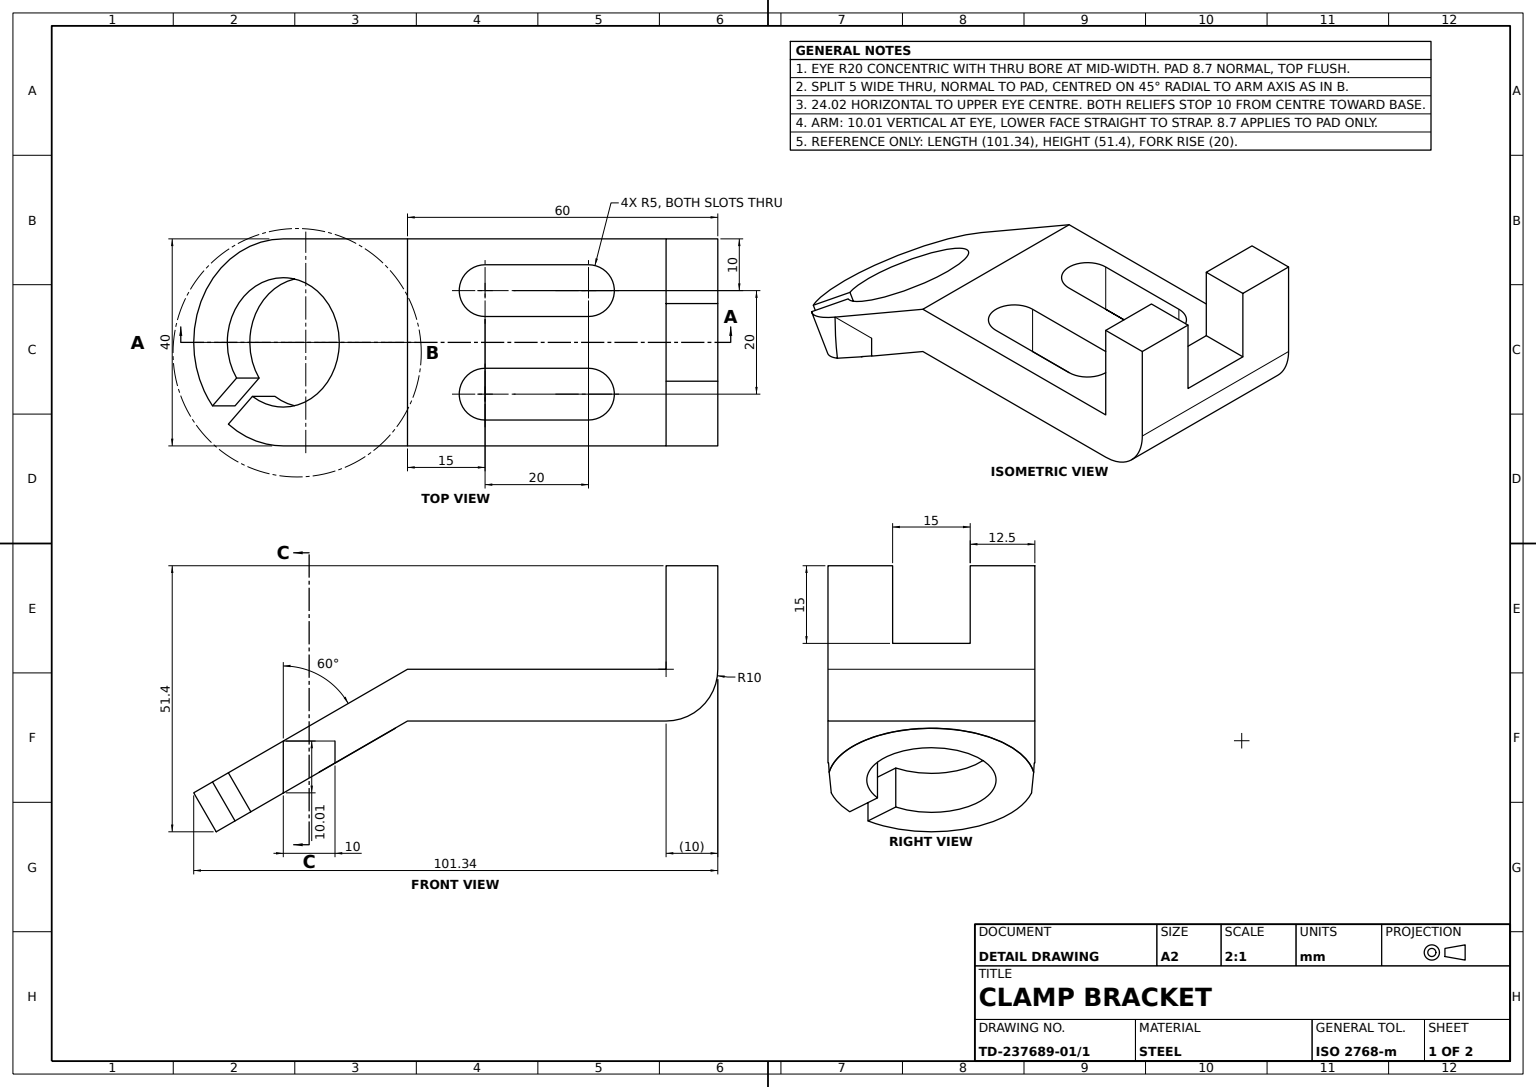
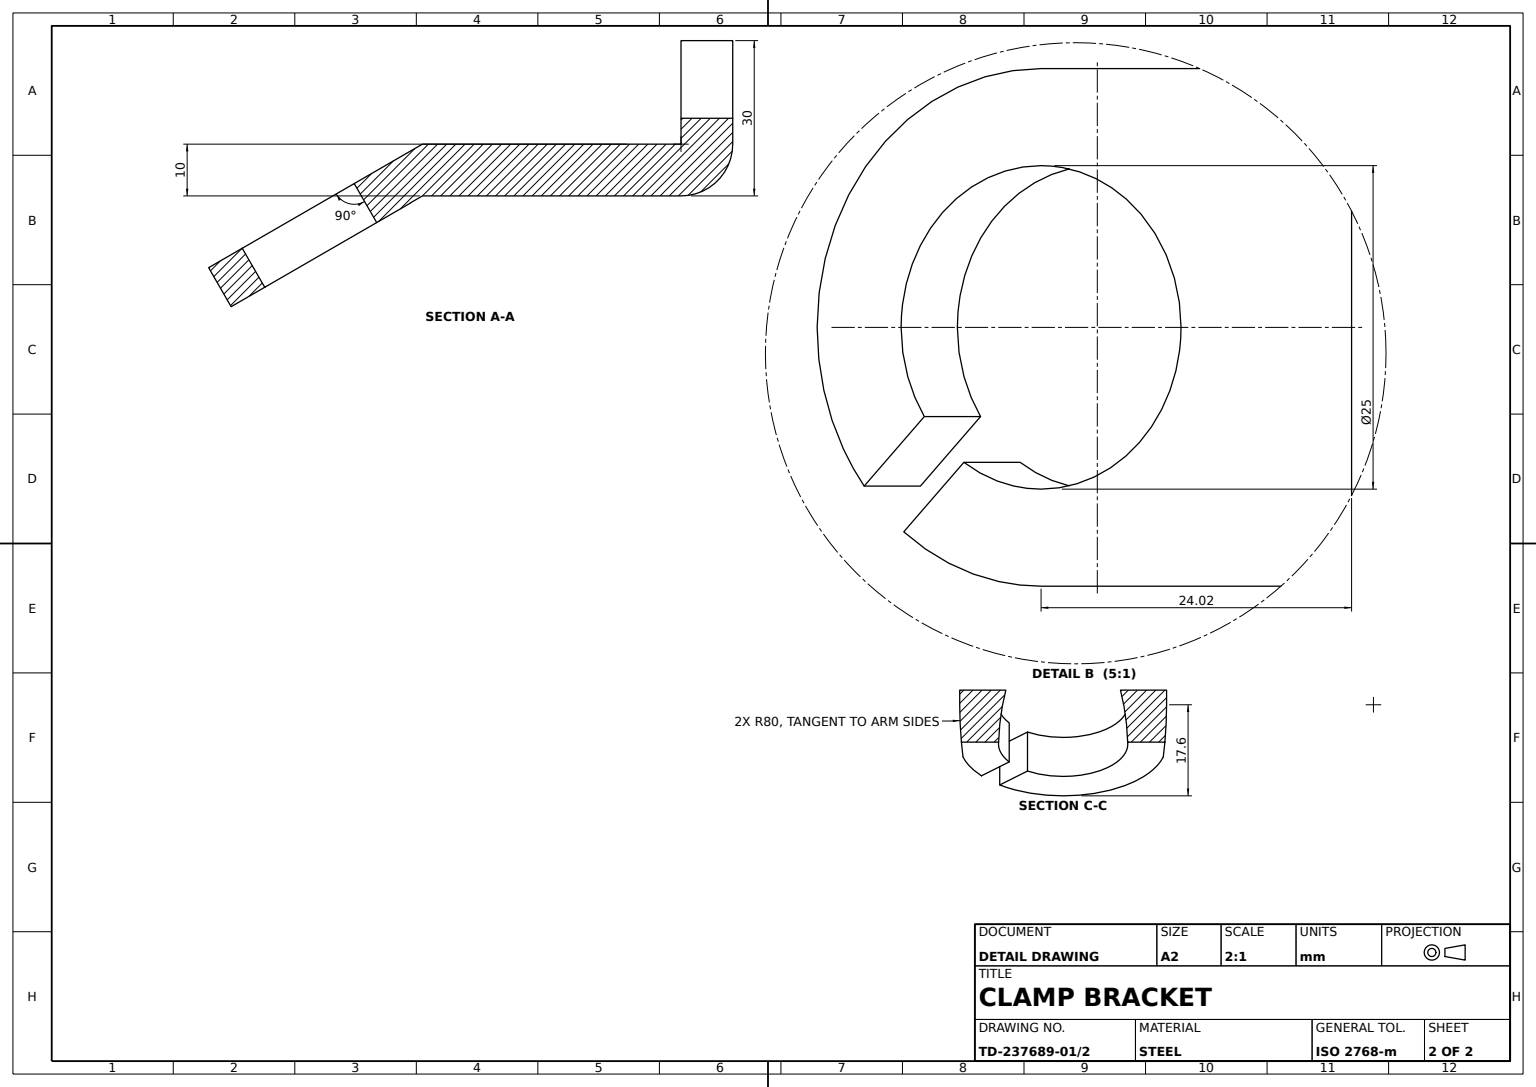
ISO-10303-21;
HEADER;
FILE_DESCRIPTION((''),'2;1');
FILE_NAME('','',(''),(''),'','','');
FILE_SCHEMA(('AUTOMOTIVE_DESIGN'));
ENDSEC;
DATA;
#1=APPLICATION_CONTEXT('');
#2=PRODUCT_CONTEXT('',#1,'mechanical');
#3=PRODUCT('','','',(#2));
#4=PRODUCT_DEFINITION_FORMATION('','',#3);
#5=PRODUCT_DEFINITION_CONTEXT('',#1,'design');
#6=PRODUCT_DEFINITION('','',#4,#5);
#7=PRODUCT_DEFINITION_SHAPE('','',#6);
#8=(LENGTH_UNIT()NAMED_UNIT(*)SI_UNIT(.MILLI.,.METRE.));
#9=(NAMED_UNIT(*)PLANE_ANGLE_UNIT()SI_UNIT($,.RADIAN.));
#10=(NAMED_UNIT(*)SI_UNIT($,.STERADIAN.)SOLID_ANGLE_UNIT());
#11=UNCERTAINTY_MEASURE_WITH_UNIT(LENGTH_MEASURE(1.E-05),#8,'distance_accuracy_value','');
#12=(GEOMETRIC_REPRESENTATION_CONTEXT(3)GLOBAL_UNCERTAINTY_ASSIGNED_CONTEXT((#11))GLOBAL_UNIT_ASSIGNED_CONTEXT((#8,#9,#10))REPRESENTATION_CONTEXT('',''));
#13=CARTESIAN_POINT('',(60.,30.,-27.5));
#14=VERTEX_POINT('',#13);
#15=CARTESIAN_POINT('',(50.,30.,-27.5));
#16=VERTEX_POINT('',#15);
#17=CARTESIAN_POINT('',(90.,30.,-27.5));
#18=DIRECTION('',(-1.,0.,0.));
#19=VECTOR('',#18,1000.);
#20=LINE('',#17,#19);
#21=EDGE_CURVE('',#14,#16,#20,.T.);
#22=ORIENTED_EDGE('',*,*,#21,.F.);
#23=CARTESIAN_POINT('',(60.,30.,-40.));
#24=VERTEX_POINT('',#23);
#25=DIRECTION('',(0.,0.,1.));
#26=VECTOR('',#25,1000.);
#27=LINE('',#23,#26);
#28=EDGE_CURVE('',#24,#14,#27,.T.);
#29=ORIENTED_EDGE('',*,*,#28,.F.);
#30=CARTESIAN_POINT('',(50.,30.,-40.));
#31=VERTEX_POINT('',#30);
#32=LINE('',#23,#19);
#33=EDGE_CURVE('',#24,#31,#32,.T.);
#34=ORIENTED_EDGE('',*,*,#33,.T.);
#35=LINE('',#30,#26);
#36=EDGE_CURVE('',#31,#16,#35,.T.);
#37=ORIENTED_EDGE('',*,*,#36,.T.);
#38=EDGE_LOOP('',(#22,#29,#34,#37));
#39=FACE_OUTER_BOUND('',#38,.T.);
#40=DIRECTION('',(0.,1.,0.));
#41=AXIS2_PLACEMENT_3D('',#23,#40,#25);
#42=PLANE('',#41);
#43=ADVANCED_FACE('',(#39),#42,.T.);
#44=CARTESIAN_POINT('',(60.,30.,-12.5));
#45=VERTEX_POINT('',#44);
#46=CARTESIAN_POINT('',(60.,15.,-12.5));
#47=VERTEX_POINT('',#46);
#48=CARTESIAN_POINT('',(60.,10.,-12.5));
#49=DIRECTION('',(0.,-1.,0.));
#50=VECTOR('',#49,1000.);
#51=LINE('',#48,#50);
#52=EDGE_CURVE('',#45,#47,#51,.T.);
#53=ORIENTED_EDGE('',*,*,#52,.T.);
#54=CARTESIAN_POINT('',(50.,15.,-12.5));
#55=VERTEX_POINT('',#54);
#56=CARTESIAN_POINT('',(90.,15.,-12.5));
#57=LINE('',#56,#19);
#58=EDGE_CURVE('',#47,#55,#57,.T.);
#59=ORIENTED_EDGE('',*,*,#58,.T.);
#60=CARTESIAN_POINT('',(50.,30.,-12.5));
#61=VERTEX_POINT('',#60);
#62=VECTOR('',#40,1000.);
#63=LINE('',#54,#62);
#64=EDGE_CURVE('',#55,#61,#63,.T.);
#65=ORIENTED_EDGE('',*,*,#64,.T.);
#66=CARTESIAN_POINT('',(90.,30.,-12.5));
#67=LINE('',#66,#19);
#68=EDGE_CURVE('',#45,#61,#67,.T.);
#69=ORIENTED_EDGE('',*,*,#68,.F.);
#70=EDGE_LOOP('',(#53,#59,#65,#69));
#71=FACE_OUTER_BOUND('',#70,.T.);
#72=DIRECTION('',(1.,0.,0.));
#73=AXIS2_PLACEMENT_3D('',#56,#25,#72);
#74=PLANE('',#73);
#75=ADVANCED_FACE('',(#71),#74,.F.);
#76=CARTESIAN_POINT('',(-17.067657,-9.860231,-39.770555));
#77=VERTEX_POINT('',#76);
#78=CARTESIAN_POINT('',(-17.040219,-9.88407,-39.768742));
#79=VERTEX_POINT('',#78);
#80=CARTESIAN_POINT('',(-17.058511,-9.868177,-39.769952));
#81=CARTESIAN_POINT('',(-17.049365,-9.876123,-39.769348));
#82=B_SPLINE_CURVE_WITH_KNOTS('',3,(#76,#80,#81,#78),.UNSPECIFIED.,.F.,.F.,(4,4),(0.00917853,0.009214903),.UNSPECIFIED.);
#83=EDGE_CURVE('',#77,#79,#82,.T.);
#84=ORIENTED_EDGE('',*,*,#83,.F.);
#85=CARTESIAN_POINT('',(-17.067657,-9.860231,-0.229445));
#86=VERTEX_POINT('',#85);
#87=CARTESIAN_POINT('',(8.925723,5.156518,-4.816157));
#88=CARTESIAN_POINT('',(8.925723,5.156518,-35.183843));
#89=(BOUNDED_CURVE()B_SPLINE_CURVE(3,(#85,#87,#88,#76),.UNSPECIFIED.,.F.,.T.)B_SPLINE_CURVE_WITH_KNOTS((4,4),(4.864008458,7.702362156),.UNSPECIFIED.)CURVE()GEOMETRIC_REPRESENTATION_ITEM()RATIONAL_B_SPLINE_CURVE((1.,0.434026152,0.434026152,1.))REPRESENTATION_ITEM(''));
#90=EDGE_CURVE('',#86,#77,#89,.T.);
#91=ORIENTED_EDGE('',*,*,#90,.F.);
#92=CARTESIAN_POINT('',(-17.040219,-9.88407,-0.231258));
#93=VERTEX_POINT('',#92);
#94=CARTESIAN_POINT('',(-17.049365,-9.876123,-0.230652));
#95=CARTESIAN_POINT('',(-17.058511,-9.868177,-0.230048));
#96=B_SPLINE_CURVE_WITH_KNOTS('',3,(#92,#94,#95,#85),.UNSPECIFIED.,.F.,.F.,(4,4),(0.,0.00003639),.UNSPECIFIED.);
#97=EDGE_CURVE('',#93,#86,#96,.T.);
#98=ORIENTED_EDGE('',*,*,#97,.F.);
#99=CARTESIAN_POINT('',(-19.666551,-11.400383,-20.));
#100=DIRECTION('',(-0.5,0.866025404,0.));
#101=DIRECTION('',(-0.866025404,-0.5,0.));
#102=AXIS2_PLACEMENT_3D('',#99,#100,#101);
#103=CIRCLE('',#102,20.);
#104=EDGE_CURVE('',#93,#79,#103,.T.);
#105=ORIENTED_EDGE('',*,*,#104,.T.);
#106=EDGE_LOOP('',(#84,#91,#98,#105));
#107=FACE_OUTER_BOUND('',#106,.T.);
#108=CYLINDRICAL_SURFACE('',#102,20.);
#109=ADVANCED_FACE('',(#107),#108,.T.);
#110=CARTESIAN_POINT('',(50.,30.,0.));
#111=VERTEX_POINT('',#110);
#112=EDGE_CURVE('',#61,#111,#35,.T.);
#113=ORIENTED_EDGE('',*,*,#112,.F.);
#114=ORIENTED_EDGE('',*,*,#64,.F.);
#115=CARTESIAN_POINT('',(50.,15.,-27.5));
#116=VERTEX_POINT('',#115);
#117=LINE('',#115,#26);
#118=EDGE_CURVE('',#116,#55,#117,.T.);
#119=ORIENTED_EDGE('',*,*,#118,.F.);
#120=LINE('',#15,#50);
#121=EDGE_CURVE('',#16,#116,#120,.T.);
#122=ORIENTED_EDGE('',*,*,#121,.F.);
#123=ORIENTED_EDGE('',*,*,#36,.F.);
#124=CARTESIAN_POINT('',(50.,10.,-40.));
#125=VERTEX_POINT('',#124);
#126=LINE('',#124,#50);
#127=EDGE_CURVE('',#31,#125,#126,.T.);
#128=ORIENTED_EDGE('',*,*,#127,.T.);
#129=CARTESIAN_POINT('',(50.,10.,0.));
#130=VERTEX_POINT('',#129);
#131=LINE('',#124,#26);
#132=EDGE_CURVE('',#125,#130,#131,.T.);
#133=ORIENTED_EDGE('',*,*,#132,.T.);
#134=LINE('',#129,#50);
#135=EDGE_CURVE('',#111,#130,#134,.T.);
#136=ORIENTED_EDGE('',*,*,#135,.F.);
#137=EDGE_LOOP('',(#113,#114,#119,#122,#123,#128,#133,#136));
#138=FACE_OUTER_BOUND('',#137,.T.);
#139=AXIS2_PLACEMENT_3D('',#124,#18,#25);
#140=PLANE('',#139);
#141=ADVANCED_FACE('',(#138),#140,.T.);
#142=CARTESIAN_POINT('',(-23.952204,-13.874706,-39.363787));
#143=VERTEX_POINT('',#142);
#144=CARTESIAN_POINT('',(-24.016551,-13.874706,-39.363787));
#145=VERTEX_POINT('',#144);
#146=CARTESIAN_POINT('',(-14.016551,-13.874706,-39.363787));
#147=LINE('',#146,#19);
#148=EDGE_CURVE('',#143,#145,#147,.T.);
#149=ORIENTED_EDGE('',*,*,#148,.F.);
#150=CARTESIAN_POINT('',(-23.952204,-13.874706,-39.378104));
#151=VERTEX_POINT('',#150);
#152=CARTESIAN_POINT('',(-23.952204,-13.874706,-20.));
#153=LINE('',#152,#26);
#154=EDGE_CURVE('',#151,#143,#153,.T.);
#155=ORIENTED_EDGE('',*,*,#154,.F.);
#156=CARTESIAN_POINT('',(-23.973661,-13.874706,-39.373358));
#157=CARTESIAN_POINT('',(-23.99511,-13.874706,-39.368586));
#158=(BOUNDED_CURVE()B_SPLINE_CURVE(3,(#150,#156,#157,#144),.UNSPECIFIED.,.F.,.T.)B_SPLINE_CURVE_WITH_KNOTS((4,4),(4.962418222,4.965295009),.UNSPECIFIED.)CURVE()GEOMETRIC_REPRESENTATION_ITEM()RATIONAL_B_SPLINE_CURVE((1.,0.99999931,0.99999931,1.))REPRESENTATION_ITEM(''));
#159=EDGE_CURVE('',#151,#145,#158,.T.);
#160=ORIENTED_EDGE('',*,*,#159,.T.);
#161=EDGE_LOOP('',(#149,#155,#160));
#162=FACE_OUTER_BOUND('',#161,.T.);
#163=CARTESIAN_POINT('',(-14.016551,-13.874706,-40.));
#164=DIRECTION('',(0.,0.,-1.));
#165=AXIS2_PLACEMENT_3D('',#163,#49,#164);
#166=PLANE('',#165);
#167=ADVANCED_FACE('',(#162),#166,.F.);
#168=CARTESIAN_POINT('',(-24.016551,-3.865962,-40.));
#169=VERTEX_POINT('',#168);
#170=CARTESIAN_POINT('',(-24.016551,-10.556136,-39.784836));
#171=CARTESIAN_POINT('',(-24.016551,-7.211136,-39.997464));
#172=B_SPLINE_CURVE_WITH_KNOTS('',3,(#144,#170,#171,#168),.UNSPECIFIED.,.F.,.F.,(4,4),(0.,1.),.UNSPECIFIED.);
#173=EDGE_CURVE('',#145,#169,#172,.T.);
#174=ORIENTED_EDGE('',*,*,#173,.T.);
#175=CARTESIAN_POINT('',(-14.016551,-3.865962,-40.));
#176=VERTEX_POINT('',#175);
#177=LINE('',#175,#19);
#178=EDGE_CURVE('',#176,#169,#177,.T.);
#179=ORIENTED_EDGE('',*,*,#178,.F.);
#180=CARTESIAN_POINT('',(-14.016551,-8.097563,-39.884793));
#181=VERTEX_POINT('',#180);
#182=CARTESIAN_POINT('',(-14.016551,-3.805302,39.999977));
#183=AXIS2_PLACEMENT_3D('',#182,#72,#164);
#184=CIRCLE('',#183,80.);
#185=EDGE_CURVE('',#181,#176,#184,.T.);
#186=ORIENTED_EDGE('',*,*,#185,.F.);
#187=CARTESIAN_POINT('',(-16.05137,-9.273107,-39.815121));
#188=CARTESIAN_POINT('',(-15.034294,-8.685527,-39.853201));
#189=(BOUNDED_CURVE()B_SPLINE_CURVE(3,(#76,#187,#188,#180),.UNSPECIFIED.,.F.,.T.)B_SPLINE_CURVE_WITH_KNOTS((4,4),(1.49503727,1.51711729),.UNSPECIFIED.)CURVE()GEOMETRIC_REPRESENTATION_ITEM()RATIONAL_B_SPLINE_CURVE((1.,0.999959373,0.999959373,1.))REPRESENTATION_ITEM(''));
#190=EDGE_CURVE('',#77,#181,#189,.T.);
#191=ORIENTED_EDGE('',*,*,#190,.F.);
#192=ORIENTED_EDGE('',*,*,#83,.T.);
#193=CARTESIAN_POINT('',(-21.654313,-12.548018,-39.532113));
#194=CARTESIAN_POINT('',(-19.349835,-11.217527,-39.667126));
#195=(BOUNDED_CURVE()B_SPLINE_CURVE(3,(#142,#193,#194,#78),.UNSPECIFIED.,.F.,.T.)B_SPLINE_CURVE_WITH_KNOTS((4,4),(1.444594034,1.494738419),.UNSPECIFIED.)CURVE()GEOMETRIC_REPRESENTATION_ITEM()RATIONAL_B_SPLINE_CURVE((1.,0.999790473,0.999790473,1.))REPRESENTATION_ITEM(''));
#196=EDGE_CURVE('',#143,#79,#195,.T.);
#197=ORIENTED_EDGE('',*,*,#196,.F.);
#198=ORIENTED_EDGE('',*,*,#148,.T.);
#199=EDGE_LOOP('',(#174,#179,#186,#191,#192,#197,#198));
#200=FACE_OUTER_BOUND('',#199,.T.);
#201=AXIS2_PLACEMENT_3D('',#182,#18,#25);
#202=CYLINDRICAL_SURFACE('',#201,80.);
#203=ADVANCED_FACE('',(#200),#202,.T.);
#204=CARTESIAN_POINT('',(35.,10.,-25.));
#205=VERTEX_POINT('',#204);
#206=CARTESIAN_POINT('',(35.,10.,-35.));
#207=VERTEX_POINT('',#206);
#208=CARTESIAN_POINT('',(35.,10.,-30.));
#209=AXIS2_PLACEMENT_3D('',#208,#40,#25);
#210=CIRCLE('',#209,5.);
#211=EDGE_CURVE('',#205,#207,#210,.T.);
#212=ORIENTED_EDGE('',*,*,#211,.T.);
#213=CARTESIAN_POINT('',(35.,0.,-35.));
#214=VERTEX_POINT('',#213);
#215=LINE('',#213,#62);
#216=EDGE_CURVE('',#214,#207,#215,.T.);
#217=ORIENTED_EDGE('',*,*,#216,.F.);
#218=CARTESIAN_POINT('',(35.,0.,-25.));
#219=VERTEX_POINT('',#218);
#220=CARTESIAN_POINT('',(35.,0.,-30.));
#221=AXIS2_PLACEMENT_3D('',#220,#40,#25);
#222=CIRCLE('',#221,5.);
#223=EDGE_CURVE('',#219,#214,#222,.T.);
#224=ORIENTED_EDGE('',*,*,#223,.F.);
#225=LINE('',#218,#62);
#226=EDGE_CURVE('',#219,#205,#225,.T.);
#227=ORIENTED_EDGE('',*,*,#226,.T.);
#228=EDGE_LOOP('',(#212,#217,#224,#227));
#229=FACE_OUTER_BOUND('',#228,.T.);
#230=CYLINDRICAL_SURFACE('',#221,5.);
#231=ADVANCED_FACE('',(#229),#230,.F.);
#232=CARTESIAN_POINT('',(-33.348871,-19.299874,-7.736552));
#233=VERTEX_POINT('',#232);
#234=CARTESIAN_POINT('',(-37.698871,-11.765453,-7.736552));
#235=VERTEX_POINT('',#234);
#236=CARTESIAN_POINT('',(-32.698871,-20.425707,-7.736552));
#237=VECTOR('',#100,1000.);
#238=LINE('',#236,#237);
#239=EDGE_CURVE('',#233,#235,#238,.T.);
#240=ORIENTED_EDGE('',*,*,#239,.F.);
#241=CARTESIAN_POINT('',(-28.697482,-16.614394,-13.107513));
#242=VERTEX_POINT('',#241);
#243=CARTESIAN_POINT('',(-21.197482,-12.284267,-21.767767));
#244=DIRECTION('',(-0.612372436,-0.353553391,0.707106781));
#245=VECTOR('',#244,1000.);
#246=LINE('',#243,#245);
#247=EDGE_CURVE('',#242,#233,#246,.T.);
#248=ORIENTED_EDGE('',*,*,#247,.F.);
#249=CARTESIAN_POINT('',(-33.047482,-9.079973,-13.107513));
#250=VERTEX_POINT('',#249);
#251=CARTESIAN_POINT('',(-28.047482,-17.740227,-13.107513));
#252=LINE('',#251,#237);
#253=EDGE_CURVE('',#242,#250,#252,.T.);
#254=ORIENTED_EDGE('',*,*,#253,.T.);
#255=LINE('',#234,#245);
#256=EDGE_CURVE('',#250,#235,#255,.T.);
#257=ORIENTED_EDGE('',*,*,#256,.T.);
#258=EDGE_LOOP('',(#240,#248,#254,#257));
#259=FACE_OUTER_BOUND('',#258,.T.);
#260=DIRECTION('',(-0.612372436,-0.353553391,-0.707106781));
#261=DIRECTION('',(-0.755928946,0.,0.654653671));
#262=AXIS2_PLACEMENT_3D('',#236,#260,#261);
#263=PLANE('',#262);
#264=ADVANCED_FACE('',(#259),#263,.F.);
#265=CARTESIAN_POINT('',(15.,10.,-5.));
#266=VERTEX_POINT('',#265);
#267=CARTESIAN_POINT('',(35.,10.,-5.));
#268=VERTEX_POINT('',#267);
#269=CARTESIAN_POINT('',(0.,10.,-5.));
#270=VECTOR('',#72,1000.);
#271=LINE('',#269,#270);
#272=EDGE_CURVE('',#266,#268,#271,.T.);
#273=ORIENTED_EDGE('',*,*,#272,.F.);
#274=CARTESIAN_POINT('',(15.,10.,-15.));
#275=VERTEX_POINT('',#274);
#276=CARTESIAN_POINT('',(15.,10.,-10.));
#277=AXIS2_PLACEMENT_3D('',#276,#40,#25);
#278=CIRCLE('',#277,5.);
#279=EDGE_CURVE('',#275,#266,#278,.T.);
#280=ORIENTED_EDGE('',*,*,#279,.F.);
#281=CARTESIAN_POINT('',(35.,10.,-15.));
#282=VERTEX_POINT('',#281);
#283=CARTESIAN_POINT('',(0.,10.,-15.));
#284=LINE('',#283,#270);
#285=EDGE_CURVE('',#275,#282,#284,.T.);
#286=ORIENTED_EDGE('',*,*,#285,.T.);
#287=CARTESIAN_POINT('',(35.,10.,-10.));
#288=AXIS2_PLACEMENT_3D('',#287,#40,#25);
#289=CIRCLE('',#288,5.);
#290=EDGE_CURVE('',#268,#282,#289,.T.);
#291=ORIENTED_EDGE('',*,*,#290,.F.);
#292=EDGE_LOOP('',(#273,#280,#286,#291));
#293=FACE_BOUND('',#292,.T.);
#294=ORIENTED_EDGE('',*,*,#132,.F.);
#295=CARTESIAN_POINT('',(0.,10.,-40.));
#296=VERTEX_POINT('',#295);
#297=LINE('',#295,#19);
#298=EDGE_CURVE('',#125,#296,#297,.T.);
#299=ORIENTED_EDGE('',*,*,#298,.T.);
#300=CARTESIAN_POINT('',(0.,10.,0.));
#301=VERTEX_POINT('',#300);
#302=LINE('',#295,#26);
#303=EDGE_CURVE('',#296,#301,#302,.T.);
#304=ORIENTED_EDGE('',*,*,#303,.T.);
#305=LINE('',#300,#19);
#306=EDGE_CURVE('',#130,#301,#305,.T.);
#307=ORIENTED_EDGE('',*,*,#306,.F.);
#308=EDGE_LOOP('',(#294,#299,#304,#307));
#309=FACE_OUTER_BOUND('',#308,.T.);
#310=ORIENTED_EDGE('',*,*,#211,.F.);
#311=CARTESIAN_POINT('',(15.,10.,-25.));
#312=VERTEX_POINT('',#311);
#313=CARTESIAN_POINT('',(0.,10.,-25.));
#314=LINE('',#313,#270);
#315=EDGE_CURVE('',#312,#205,#314,.T.);
#316=ORIENTED_EDGE('',*,*,#315,.F.);
#317=CARTESIAN_POINT('',(15.,10.,-35.));
#318=VERTEX_POINT('',#317);
#319=CARTESIAN_POINT('',(15.,10.,-30.));
#320=AXIS2_PLACEMENT_3D('',#319,#40,#25);
#321=CIRCLE('',#320,5.);
#322=EDGE_CURVE('',#318,#312,#321,.T.);
#323=ORIENTED_EDGE('',*,*,#322,.F.);
#324=CARTESIAN_POINT('',(0.,10.,-35.));
#325=LINE('',#324,#270);
#326=EDGE_CURVE('',#318,#207,#325,.T.);
#327=ORIENTED_EDGE('',*,*,#326,.T.);
#328=EDGE_LOOP('',(#310,#316,#323,#327));
#329=FACE_BOUND('',#328,.T.);
#330=AXIS2_PLACEMENT_3D('',#295,#40,#25);
#331=PLANE('',#330);
#332=ADVANCED_FACE('',(#293,#309,#329),#331,.T.);
#333=CARTESIAN_POINT('',(15.,0.,-15.));
#334=VERTEX_POINT('',#333);
#335=CARTESIAN_POINT('',(35.,0.,-15.));
#336=VERTEX_POINT('',#335);
#337=CARTESIAN_POINT('',(0.,0.,-15.));
#338=LINE('',#337,#270);
#339=EDGE_CURVE('',#334,#336,#338,.T.);
#340=ORIENTED_EDGE('',*,*,#339,.T.);
#341=LINE('',#335,#62);
#342=EDGE_CURVE('',#336,#282,#341,.T.);
#343=ORIENTED_EDGE('',*,*,#342,.T.);
#344=ORIENTED_EDGE('',*,*,#285,.F.);
#345=LINE('',#333,#62);
#346=EDGE_CURVE('',#334,#275,#345,.T.);
#347=ORIENTED_EDGE('',*,*,#346,.F.);
#348=EDGE_LOOP('',(#340,#343,#344,#347));
#349=FACE_OUTER_BOUND('',#348,.T.);
#350=AXIS2_PLACEMENT_3D('',#337,#25,#72);
#351=PLANE('',#350);
#352=ADVANCED_FACE('',(#349),#351,.T.);
#353=CARTESIAN_POINT('',(-34.637009,-9.997687,-4.201018));
#354=VERTEX_POINT('',#353);
#355=CARTESIAN_POINT('',(-24.016551,-3.865962,0.));
#356=VERTEX_POINT('',#355);
#357=CARTESIAN_POINT('',(-24.016551,-3.865962,-20.));
#358=AXIS2_PLACEMENT_3D('',#357,#100,#101);
#359=CIRCLE('',#358,20.);
#360=EDGE_CURVE('',#354,#356,#359,.T.);
#361=ORIENTED_EDGE('',*,*,#360,.F.);
#362=CARTESIAN_POINT('',(-30.287009,-17.532108,-4.201018));
#363=VERTEX_POINT('',#362);
#364=CARTESIAN_POINT('',(-29.637009,-18.657941,-4.201018));
#365=LINE('',#364,#237);
#366=EDGE_CURVE('',#363,#354,#365,.T.);
#367=ORIENTED_EDGE('',*,*,#366,.F.);
#368=CARTESIAN_POINT('',(-23.952204,-13.874706,-0.621896));
#369=VERTEX_POINT('',#368);
#370=EDGE_CURVE('',#363,#369,#103,.T.);
#371=ORIENTED_EDGE('',*,*,#370,.T.);
#372=CARTESIAN_POINT('',(-24.016551,-13.874706,-0.636213));
#373=VERTEX_POINT('',#372);
#374=CARTESIAN_POINT('',(-23.99511,-13.874706,-0.631414));
#375=CARTESIAN_POINT('',(-23.973661,-13.874706,-0.626642));
#376=(BOUNDED_CURVE()B_SPLINE_CURVE(3,(#372,#374,#375,#368),.UNSPECIFIED.,.F.,.T.)B_SPLINE_CURVE_WITH_KNOTS((4,4),(1.317890298,1.320767086),.UNSPECIFIED.)CURVE()GEOMETRIC_REPRESENTATION_ITEM()RATIONAL_B_SPLINE_CURVE((1.,0.99999931,0.99999931,1.))REPRESENTATION_ITEM(''));
#377=EDGE_CURVE('',#373,#369,#376,.T.);
#378=ORIENTED_EDGE('',*,*,#377,.F.);
#379=CARTESIAN_POINT('',(-24.016551,-7.211136,-0.002536));
#380=CARTESIAN_POINT('',(-24.016551,-10.556136,-0.215164));
#381=B_SPLINE_CURVE_WITH_KNOTS('',3,(#355,#379,#380,#372),.UNSPECIFIED.,.F.,.F.,(4,4),(0.,1.),.UNSPECIFIED.);
#382=EDGE_CURVE('',#356,#373,#381,.T.);
#383=ORIENTED_EDGE('',*,*,#382,.F.);
#384=EDGE_LOOP('',(#361,#367,#371,#378,#383));
#385=FACE_OUTER_BOUND('',#384,.T.);
#386=ADVANCED_FACE('',(#385),#108,.T.);
#387=ORIENTED_EDGE('',*,*,#366,.T.);
#388=CARTESIAN_POINT('',(-29.98562,-7.312206,-9.571979));
#389=VERTEX_POINT('',#388);
#390=DIRECTION('',(0.612372436,0.353553391,-0.707106781));
#391=VECTOR('',#390,1000.);
#392=LINE('',#388,#391);
#393=EDGE_CURVE('',#354,#389,#392,.T.);
#394=ORIENTED_EDGE('',*,*,#393,.T.);
#395=CARTESIAN_POINT('',(-25.63562,-14.846627,-9.571979));
#396=VERTEX_POINT('',#395);
#397=CARTESIAN_POINT('',(-24.98562,-15.97246,-9.571979));
#398=LINE('',#397,#237);
#399=EDGE_CURVE('',#396,#389,#398,.T.);
#400=ORIENTED_EDGE('',*,*,#399,.F.);
#401=CARTESIAN_POINT('',(-18.13562,-10.5165,-18.232233));
#402=LINE('',#401,#391);
#403=EDGE_CURVE('',#363,#396,#402,.T.);
#404=ORIENTED_EDGE('',*,*,#403,.F.);
#405=EDGE_LOOP('',(#387,#394,#400,#404));
#406=FACE_OUTER_BOUND('',#405,.T.);
#407=DIRECTION('',(0.612372436,0.353553391,0.707106781));
#408=DIRECTION('',(0.755928946,0.,-0.654653671));
#409=AXIS2_PLACEMENT_3D('',#397,#407,#408);
#410=PLANE('',#409);
#411=ADVANCED_FACE('',(#406),#410,.F.);
#412=CARTESIAN_POINT('',(-30.491869,-17.650383,-20.));
#413=VERTEX_POINT('',#412);
#414=CARTESIAN_POINT('',(-34.841869,-10.115962,-20.));
#415=VERTEX_POINT('',#414);
#416=CARTESIAN_POINT('',(-29.841869,-18.776216,-20.));
#417=LINE('',#416,#237);
#418=EDGE_CURVE('',#413,#415,#417,.T.);
#419=ORIENTED_EDGE('',*,*,#418,.F.);
#420=CARTESIAN_POINT('',(-8.841234,-5.150383,-20.));
#421=VERTEX_POINT('',#420);
#422=CIRCLE('',#102,12.5);
#423=EDGE_CURVE('',#421,#413,#422,.T.);
#424=ORIENTED_EDGE('',*,*,#423,.F.);
#425=CARTESIAN_POINT('',(-13.191234,2.384038,-20.));
#426=VERTEX_POINT('',#425);
#427=CARTESIAN_POINT('',(-8.191234,-6.276216,-20.));
#428=LINE('',#427,#237);
#429=EDGE_CURVE('',#421,#426,#428,.T.);
#430=ORIENTED_EDGE('',*,*,#429,.T.);
#431=CIRCLE('',#358,12.5);
#432=EDGE_CURVE('',#426,#415,#431,.T.);
#433=ORIENTED_EDGE('',*,*,#432,.T.);
#434=EDGE_LOOP('',(#419,#424,#430,#433));
#435=FACE_OUTER_BOUND('',#434,.T.);
#436=CARTESIAN_POINT('',(-19.016551,-12.526216,-20.));
#437=AXIS2_PLACEMENT_3D('',#436,#100,#101);
#438=CYLINDRICAL_SURFACE('',#437,12.5);
#439=ADVANCED_FACE('',(#435),#438,.F.);
#440=CARTESIAN_POINT('',(15.,0.,-5.));
#441=VERTEX_POINT('',#440);
#442=CARTESIAN_POINT('',(15.,0.,-10.));
#443=AXIS2_PLACEMENT_3D('',#442,#40,#25);
#444=CIRCLE('',#443,5.);
#445=EDGE_CURVE('',#334,#441,#444,.T.);
#446=ORIENTED_EDGE('',*,*,#445,.F.);
#447=ORIENTED_EDGE('',*,*,#346,.T.);
#448=ORIENTED_EDGE('',*,*,#279,.T.);
#449=LINE('',#440,#62);
#450=EDGE_CURVE('',#441,#266,#449,.T.);
#451=ORIENTED_EDGE('',*,*,#450,.F.);
#452=EDGE_LOOP('',(#446,#447,#448,#451));
#453=FACE_OUTER_BOUND('',#452,.T.);
#454=CYLINDRICAL_SURFACE('',#443,5.);
#455=ADVANCED_FACE('',(#453),#454,.F.);
#456=ORIENTED_EDGE('',*,*,#377,.T.);
#457=CARTESIAN_POINT('',(-23.952204,-13.874706,-0.636213));
#458=VERTEX_POINT('',#457);
#459=EDGE_CURVE('',#458,#369,#153,.T.);
#460=ORIENTED_EDGE('',*,*,#459,.F.);
#461=CARTESIAN_POINT('',(-14.016551,-13.874706,-0.636213));
#462=LINE('',#461,#19);
#463=EDGE_CURVE('',#458,#373,#462,.T.);
#464=ORIENTED_EDGE('',*,*,#463,.T.);
#465=EDGE_LOOP('',(#456,#460,#464));
#466=FACE_OUTER_BOUND('',#465,.T.);
#467=AXIS2_PLACEMENT_3D('',#461,#49,#164);
#468=PLANE('',#467);
#469=ADVANCED_FACE('',(#466),#468,.F.);
#470=CARTESIAN_POINT('',(60.,30.,0.));
#471=VERTEX_POINT('',#470);
#472=LINE('',#470,#19);
#473=EDGE_CURVE('',#471,#111,#472,.T.);
#474=ORIENTED_EDGE('',*,*,#473,.F.);
#475=EDGE_CURVE('',#45,#471,#27,.T.);
#476=ORIENTED_EDGE('',*,*,#475,.F.);
#477=ORIENTED_EDGE('',*,*,#68,.T.);
#478=ORIENTED_EDGE('',*,*,#112,.T.);
#479=EDGE_LOOP('',(#474,#476,#477,#478));
#480=FACE_OUTER_BOUND('',#479,.T.);
#481=ADVANCED_FACE('',(#480),#42,.T.);
#482=CARTESIAN_POINT('',(-14.016551,-8.097563,0.));
#483=VERTEX_POINT('',#482);
#484=CARTESIAN_POINT('',(-14.016551,-8.097563,-0.115207));
#485=VERTEX_POINT('',#484);
#486=CARTESIAN_POINT('',(-14.016551,-8.097563,-40.));
#487=VECTOR('',#164,1000.);
#488=LINE('',#486,#487);
#489=EDGE_CURVE('',#483,#485,#488,.T.);
#490=ORIENTED_EDGE('',*,*,#489,.T.);
#491=CARTESIAN_POINT('',(-15.034294,-8.685527,-0.146799));
#492=CARTESIAN_POINT('',(-16.05137,-9.273107,-0.184879));
#493=(BOUNDED_CURVE()B_SPLINE_CURVE(3,(#484,#491,#492,#85),.UNSPECIFIED.,.F.,.T.)B_SPLINE_CURVE_WITH_KNOTS((4,4),(4.766068017,4.788148037),.UNSPECIFIED.)CURVE()GEOMETRIC_REPRESENTATION_ITEM()RATIONAL_B_SPLINE_CURVE((1.,0.999959373,0.999959373,1.))REPRESENTATION_ITEM(''));
#494=EDGE_CURVE('',#485,#86,#493,.T.);
#495=ORIENTED_EDGE('',*,*,#494,.T.);
#496=ORIENTED_EDGE('',*,*,#90,.T.);
#497=ORIENTED_EDGE('',*,*,#190,.T.);
#498=VERTEX_POINT('',#486);
#499=EDGE_CURVE('',#181,#498,#488,.T.);
#500=ORIENTED_EDGE('',*,*,#499,.T.);
#501=CARTESIAN_POINT('',(0.,0.,-40.));
#502=VERTEX_POINT('',#501);
#503=DIRECTION('',(-0.865888863,-0.50023642,0.));
#504=VECTOR('',#503,1000.);
#505=LINE('',#501,#504);
#506=EDGE_CURVE('',#502,#498,#505,.T.);
#507=ORIENTED_EDGE('',*,*,#506,.F.);
#508=CARTESIAN_POINT('',(0.,0.,0.));
#509=VERTEX_POINT('',#508);
#510=LINE('',#501,#26);
#511=EDGE_CURVE('',#502,#509,#510,.T.);
#512=ORIENTED_EDGE('',*,*,#511,.T.);
#513=LINE('',#508,#504);
#514=EDGE_CURVE('',#509,#483,#513,.T.);
#515=ORIENTED_EDGE('',*,*,#514,.T.);
#516=EDGE_LOOP('',(#490,#495,#496,#497,#500,#507,#512,#515));
#517=FACE_OUTER_BOUND('',#516,.T.);
#518=DIRECTION('',(-0.50023642,0.865888863,0.));
#519=AXIS2_PLACEMENT_3D('',#501,#518,#503);
#520=PLANE('',#519);
#521=ADVANCED_FACE('',(#517),#520,.F.);
#522=CARTESIAN_POINT('',(35.,0.,-5.));
#523=VERTEX_POINT('',#522);
#524=LINE('',#522,#62);
#525=EDGE_CURVE('',#523,#268,#524,.T.);
#526=ORIENTED_EDGE('',*,*,#525,.F.);
#527=CARTESIAN_POINT('',(0.,0.,-5.));
#528=LINE('',#527,#270);
#529=EDGE_CURVE('',#441,#523,#528,.T.);
#530=ORIENTED_EDGE('',*,*,#529,.F.);
#531=ORIENTED_EDGE('',*,*,#450,.T.);
#532=ORIENTED_EDGE('',*,*,#272,.T.);
#533=EDGE_LOOP('',(#526,#530,#531,#532));
#534=FACE_OUTER_BOUND('',#533,.T.);
#535=AXIS2_PLACEMENT_3D('',#527,#25,#72);
#536=PLANE('',#535);
#537=ADVANCED_FACE('',(#534),#536,.F.);
#538=ORIENTED_EDGE('',*,*,#21,.T.);
#539=ORIENTED_EDGE('',*,*,#121,.T.);
#540=CARTESIAN_POINT('',(60.,15.,-27.5));
#541=VERTEX_POINT('',#540);
#542=CARTESIAN_POINT('',(90.,15.,-27.5));
#543=LINE('',#542,#19);
#544=EDGE_CURVE('',#541,#116,#543,.T.);
#545=ORIENTED_EDGE('',*,*,#544,.F.);
#546=CARTESIAN_POINT('',(60.,10.,-27.5));
#547=LINE('',#546,#62);
#548=EDGE_CURVE('',#541,#14,#547,.T.);
#549=ORIENTED_EDGE('',*,*,#548,.T.);
#550=EDGE_LOOP('',(#538,#539,#545,#549));
#551=FACE_OUTER_BOUND('',#550,.T.);
#552=AXIS2_PLACEMENT_3D('',#17,#164,#18);
#553=PLANE('',#552);
#554=ADVANCED_FACE('',(#551),#553,.F.);
#555=EDGE_CURVE('',#413,#242,#422,.T.);
#556=ORIENTED_EDGE('',*,*,#555,.F.);
#557=ORIENTED_EDGE('',*,*,#418,.T.);
#558=EDGE_CURVE('',#415,#250,#431,.T.);
#559=ORIENTED_EDGE('',*,*,#558,.T.);
#560=ORIENTED_EDGE('',*,*,#253,.F.);
#561=EDGE_LOOP('',(#556,#557,#559,#560));
#562=FACE_OUTER_BOUND('',#561,.T.);
#563=ADVANCED_FACE('',(#562),#438,.F.);
#564=ORIENTED_EDGE('',*,*,#514,.F.);
#565=CARTESIAN_POINT('',(50.,0.,0.));
#566=VERTEX_POINT('',#565);
#567=LINE('',#508,#270);
#568=EDGE_CURVE('',#509,#566,#567,.T.);
#569=ORIENTED_EDGE('',*,*,#568,.T.);
#570=CARTESIAN_POINT('',(60.,10.,0.));
#571=VERTEX_POINT('',#570);
#572=AXIS2_PLACEMENT_3D('',#129,#25,#72);
#573=CIRCLE('',#572,10.);
#574=EDGE_CURVE('',#566,#571,#573,.T.);
#575=ORIENTED_EDGE('',*,*,#574,.T.);
#576=LINE('',#570,#62);
#577=EDGE_CURVE('',#571,#471,#576,.T.);
#578=ORIENTED_EDGE('',*,*,#577,.T.);
#579=ORIENTED_EDGE('',*,*,#473,.T.);
#580=ORIENTED_EDGE('',*,*,#135,.T.);
#581=ORIENTED_EDGE('',*,*,#306,.T.);
#582=CARTESIAN_POINT('',(-4.330127,7.5,0.));
#583=VECTOR('',#101,1000.);
#584=LINE('',#582,#583);
#585=EDGE_CURVE('',#301,#356,#584,.T.);
#586=ORIENTED_EDGE('',*,*,#585,.T.);
#587=CARTESIAN_POINT('',(-14.016551,-3.865962,0.));
#588=VERTEX_POINT('',#587);
#589=LINE('',#587,#19);
#590=EDGE_CURVE('',#588,#356,#589,.T.);
#591=ORIENTED_EDGE('',*,*,#590,.F.);
#592=CARTESIAN_POINT('',(-14.016551,-13.874706,0.));
#593=LINE('',#592,#62);
#594=EDGE_CURVE('',#483,#588,#593,.T.);
#595=ORIENTED_EDGE('',*,*,#594,.F.);
#596=EDGE_LOOP('',(#564,#569,#575,#578,#579,#580,#581,#586,#591,#595));
#597=FACE_OUTER_BOUND('',#596,.T.);
#598=PLANE('',#572);
#599=ADVANCED_FACE('',(#597),#598,.T.);
#600=CARTESIAN_POINT('',(15.,0.,-35.));
#601=VERTEX_POINT('',#600);
#602=CARTESIAN_POINT('',(0.,0.,-35.));
#603=LINE('',#602,#270);
#604=EDGE_CURVE('',#601,#214,#603,.T.);
#605=ORIENTED_EDGE('',*,*,#604,.F.);
#606=CARTESIAN_POINT('',(15.,0.,-25.));
#607=VERTEX_POINT('',#606);
#608=CARTESIAN_POINT('',(15.,0.,-30.));
#609=AXIS2_PLACEMENT_3D('',#608,#40,#25);
#610=CIRCLE('',#609,5.);
#611=EDGE_CURVE('',#601,#607,#610,.T.);
#612=ORIENTED_EDGE('',*,*,#611,.T.);
#613=CARTESIAN_POINT('',(0.,0.,-25.));
#614=LINE('',#613,#270);
#615=EDGE_CURVE('',#607,#219,#614,.T.);
#616=ORIENTED_EDGE('',*,*,#615,.T.);
#617=ORIENTED_EDGE('',*,*,#223,.T.);
#618=EDGE_LOOP('',(#605,#612,#616,#617));
#619=FACE_BOUND('',#618,.T.);
#620=CARTESIAN_POINT('',(35.,0.,-10.));
#621=AXIS2_PLACEMENT_3D('',#620,#40,#25);
#622=CIRCLE('',#621,5.);
#623=EDGE_CURVE('',#523,#336,#622,.T.);
#624=ORIENTED_EDGE('',*,*,#623,.T.);
#625=ORIENTED_EDGE('',*,*,#339,.F.);
#626=ORIENTED_EDGE('',*,*,#445,.T.);
#627=ORIENTED_EDGE('',*,*,#529,.T.);
#628=EDGE_LOOP('',(#624,#625,#626,#627));
#629=FACE_BOUND('',#628,.T.);
#630=CARTESIAN_POINT('',(50.,0.,-40.));
#631=VERTEX_POINT('',#630);
#632=LINE('',#630,#26);
#633=EDGE_CURVE('',#631,#566,#632,.T.);
#634=ORIENTED_EDGE('',*,*,#633,.T.);
#635=ORIENTED_EDGE('',*,*,#568,.F.);
#636=ORIENTED_EDGE('',*,*,#511,.F.);
#637=LINE('',#501,#270);
#638=EDGE_CURVE('',#502,#631,#637,.T.);
#639=ORIENTED_EDGE('',*,*,#638,.T.);
#640=EDGE_LOOP('',(#634,#635,#636,#639));
#641=FACE_OUTER_BOUND('',#640,.T.);
#642=AXIS2_PLACEMENT_3D('',#501,#49,#164);
#643=PLANE('',#642);
#644=ADVANCED_FACE('',(#619,#629,#641),#643,.T.);
#645=CARTESIAN_POINT('',(-41.337059,-13.865962,-20.));
#646=VERTEX_POINT('',#645);
#647=EDGE_CURVE('',#169,#646,#359,.T.);
#648=ORIENTED_EDGE('',*,*,#647,.F.);
#649=ORIENTED_EDGE('',*,*,#173,.F.);
#650=ORIENTED_EDGE('',*,*,#159,.F.);
#651=CARTESIAN_POINT('',(-36.987059,-21.400383,-20.));
#652=VERTEX_POINT('',#651);
#653=EDGE_CURVE('',#151,#652,#103,.T.);
#654=ORIENTED_EDGE('',*,*,#653,.T.);
#655=LINE('',#651,#237);
#656=EDGE_CURVE('',#652,#646,#655,.T.);
#657=ORIENTED_EDGE('',*,*,#656,.T.);
#658=EDGE_LOOP('',(#648,#649,#650,#654,#657));
#659=FACE_OUTER_BOUND('',#658,.T.);
#660=ADVANCED_FACE('',(#659),#108,.T.);
#661=LINE('',#163,#50);
#662=EDGE_CURVE('',#176,#498,#661,.T.);
#663=ORIENTED_EDGE('',*,*,#662,.T.);
#664=ORIENTED_EDGE('',*,*,#499,.F.);
#665=ORIENTED_EDGE('',*,*,#185,.T.);
#666=EDGE_LOOP('',(#663,#664,#665));
#667=FACE_OUTER_BOUND('',#666,.T.);
#668=PLANE('',#183);
#669=ADVANCED_FACE('',(#667),#668,.F.);
#670=ORIENTED_EDGE('',*,*,#326,.F.);
#671=LINE('',#600,#62);
#672=EDGE_CURVE('',#601,#318,#671,.T.);
#673=ORIENTED_EDGE('',*,*,#672,.F.);
#674=ORIENTED_EDGE('',*,*,#604,.T.);
#675=ORIENTED_EDGE('',*,*,#216,.T.);
#676=EDGE_LOOP('',(#670,#673,#674,#675));
#677=FACE_OUTER_BOUND('',#676,.T.);
#678=AXIS2_PLACEMENT_3D('',#602,#25,#72);
#679=PLANE('',#678);
#680=ADVANCED_FACE('',(#677),#679,.T.);
#681=ORIENTED_EDGE('',*,*,#239,.T.);
#682=EDGE_CURVE('',#646,#235,#359,.T.);
#683=ORIENTED_EDGE('',*,*,#682,.F.);
#684=ORIENTED_EDGE('',*,*,#656,.F.);
#685=EDGE_CURVE('',#652,#233,#103,.T.);
#686=ORIENTED_EDGE('',*,*,#685,.T.);
#687=EDGE_LOOP('',(#681,#683,#684,#686));
#688=FACE_OUTER_BOUND('',#687,.T.);
#689=ADVANCED_FACE('',(#688),#108,.T.);
#690=ORIENTED_EDGE('',*,*,#594,.T.);
#691=CARTESIAN_POINT('',(-14.016551,-3.805302,-79.999977));
#692=AXIS2_PLACEMENT_3D('',#691,#72,#164);
#693=CIRCLE('',#692,80.);
#694=EDGE_CURVE('',#588,#485,#693,.T.);
#695=ORIENTED_EDGE('',*,*,#694,.T.);
#696=ORIENTED_EDGE('',*,*,#489,.F.);
#697=EDGE_LOOP('',(#690,#695,#696));
#698=FACE_OUTER_BOUND('',#697,.T.);
#699=PLANE('',#692);
#700=ADVANCED_FACE('',(#698),#699,.F.);
#701=ORIENTED_EDGE('',*,*,#544,.T.);
#702=ORIENTED_EDGE('',*,*,#118,.T.);
#703=ORIENTED_EDGE('',*,*,#58,.F.);
#704=CARTESIAN_POINT('',(60.,15.,-40.));
#705=LINE('',#704,#487);
#706=EDGE_CURVE('',#47,#541,#705,.T.);
#707=ORIENTED_EDGE('',*,*,#706,.T.);
#708=EDGE_LOOP('',(#701,#702,#703,#707));
#709=FACE_OUTER_BOUND('',#708,.T.);
#710=AXIS2_PLACEMENT_3D('',#542,#49,#164);
#711=PLANE('',#710);
#712=ADVANCED_FACE('',(#709),#711,.F.);
#713=ORIENTED_EDGE('',*,*,#647,.T.);
#714=ORIENTED_EDGE('',*,*,#682,.T.);
#715=ORIENTED_EDGE('',*,*,#256,.F.);
#716=ORIENTED_EDGE('',*,*,#558,.F.);
#717=ORIENTED_EDGE('',*,*,#432,.F.);
#718=EDGE_CURVE('',#389,#426,#431,.T.);
#719=ORIENTED_EDGE('',*,*,#718,.F.);
#720=ORIENTED_EDGE('',*,*,#393,.F.);
#721=ORIENTED_EDGE('',*,*,#360,.T.);
#722=ORIENTED_EDGE('',*,*,#585,.F.);
#723=ORIENTED_EDGE('',*,*,#303,.F.);
#724=CARTESIAN_POINT('',(-4.330127,7.5,-40.));
#725=LINE('',#724,#583);
#726=EDGE_CURVE('',#296,#169,#725,.T.);
#727=ORIENTED_EDGE('',*,*,#726,.T.);
#728=EDGE_LOOP('',(#713,#714,#715,#716,#717,#719,#720,#721,#722,#723,#727));
#729=FACE_OUTER_BOUND('',#728,.T.);
#730=AXIS2_PLACEMENT_3D('',#724,#100,#101);
#731=PLANE('',#730);
#732=ADVANCED_FACE('',(#729),#731,.T.);
#733=ORIENTED_EDGE('',*,*,#459,.T.);
#734=ORIENTED_EDGE('',*,*,#370,.F.);
#735=ORIENTED_EDGE('',*,*,#403,.T.);
#736=EDGE_CURVE('',#396,#421,#422,.T.);
#737=ORIENTED_EDGE('',*,*,#736,.T.);
#738=ORIENTED_EDGE('',*,*,#423,.T.);
#739=ORIENTED_EDGE('',*,*,#555,.T.);
#740=ORIENTED_EDGE('',*,*,#247,.T.);
#741=ORIENTED_EDGE('',*,*,#685,.F.);
#742=ORIENTED_EDGE('',*,*,#653,.F.);
#743=ORIENTED_EDGE('',*,*,#154,.T.);
#744=ORIENTED_EDGE('',*,*,#196,.T.);
#745=ORIENTED_EDGE('',*,*,#104,.F.);
#746=CARTESIAN_POINT('',(-19.349835,-11.217527,-0.332874));
#747=CARTESIAN_POINT('',(-21.654313,-12.548018,-0.467887));
#748=(BOUNDED_CURVE()B_SPLINE_CURVE(3,(#92,#746,#747,#457),.UNSPECIFIED.,.F.,.T.)B_SPLINE_CURVE_WITH_KNOTS((4,4),(4.788446888,4.838591273),.UNSPECIFIED.)CURVE()GEOMETRIC_REPRESENTATION_ITEM()RATIONAL_B_SPLINE_CURVE((1.,0.999790473,0.999790473,1.))REPRESENTATION_ITEM(''));
#749=EDGE_CURVE('',#93,#458,#748,.T.);
#750=ORIENTED_EDGE('',*,*,#749,.T.);
#751=EDGE_LOOP('',(#733,#734,#735,#737,#738,#739,#740,#741,#742,#743,#744,#745,#750));
#752=FACE_OUTER_BOUND('',#751,.T.);
#753=PLANE('',#102);
#754=ADVANCED_FACE('',(#752),#753,.F.);
#755=CARTESIAN_POINT('',(60.,10.,-40.));
#756=VERTEX_POINT('',#755);
#757=AXIS2_PLACEMENT_3D('',#124,#25,#72);
#758=CIRCLE('',#757,10.);
#759=EDGE_CURVE('',#631,#756,#758,.T.);
#760=ORIENTED_EDGE('',*,*,#759,.T.);
#761=LINE('',#755,#26);
#762=EDGE_CURVE('',#756,#571,#761,.T.);
#763=ORIENTED_EDGE('',*,*,#762,.T.);
#764=ORIENTED_EDGE('',*,*,#574,.F.);
#765=ORIENTED_EDGE('',*,*,#633,.F.);
#766=EDGE_LOOP('',(#760,#763,#764,#765));
#767=FACE_OUTER_BOUND('',#766,.T.);
#768=CYLINDRICAL_SURFACE('',#757,10.);
#769=ADVANCED_FACE('',(#767),#768,.T.);
#770=ORIENTED_EDGE('',*,*,#226,.F.);
#771=ORIENTED_EDGE('',*,*,#615,.F.);
#772=LINE('',#606,#62);
#773=EDGE_CURVE('',#607,#312,#772,.T.);
#774=ORIENTED_EDGE('',*,*,#773,.T.);
#775=ORIENTED_EDGE('',*,*,#315,.T.);
#776=EDGE_LOOP('',(#770,#771,#774,#775));
#777=FACE_OUTER_BOUND('',#776,.T.);
#778=AXIS2_PLACEMENT_3D('',#613,#25,#72);
#779=PLANE('',#778);
#780=ADVANCED_FACE('',(#777),#779,.F.);
#781=ORIENTED_EDGE('',*,*,#322,.T.);
#782=ORIENTED_EDGE('',*,*,#773,.F.);
#783=ORIENTED_EDGE('',*,*,#611,.F.);
#784=ORIENTED_EDGE('',*,*,#672,.T.);
#785=EDGE_LOOP('',(#781,#782,#783,#784));
#786=FACE_OUTER_BOUND('',#785,.T.);
#787=CYLINDRICAL_SURFACE('',#609,5.);
#788=ADVANCED_FACE('',(#786),#787,.F.);
#789=ORIENTED_EDGE('',*,*,#548,.F.);
#790=ORIENTED_EDGE('',*,*,#706,.F.);
#791=ORIENTED_EDGE('',*,*,#52,.F.);
#792=ORIENTED_EDGE('',*,*,#475,.T.);
#793=ORIENTED_EDGE('',*,*,#577,.F.);
#794=ORIENTED_EDGE('',*,*,#762,.F.);
#795=LINE('',#755,#62);
#796=EDGE_CURVE('',#756,#24,#795,.T.);
#797=ORIENTED_EDGE('',*,*,#796,.T.);
#798=ORIENTED_EDGE('',*,*,#28,.T.);
#799=EDGE_LOOP('',(#789,#790,#791,#792,#793,#794,#797,#798));
#800=FACE_OUTER_BOUND('',#799,.T.);
#801=AXIS2_PLACEMENT_3D('',#755,#72,#164);
#802=PLANE('',#801);
#803=ADVANCED_FACE('',(#800),#802,.T.);
#804=ORIENTED_EDGE('',*,*,#525,.T.);
#805=ORIENTED_EDGE('',*,*,#290,.T.);
#806=ORIENTED_EDGE('',*,*,#342,.F.);
#807=ORIENTED_EDGE('',*,*,#623,.F.);
#808=EDGE_LOOP('',(#804,#805,#806,#807));
#809=FACE_OUTER_BOUND('',#808,.T.);
#810=CYLINDRICAL_SURFACE('',#621,5.);
#811=ADVANCED_FACE('',(#809),#810,.F.);
#812=ORIENTED_EDGE('',*,*,#796,.F.);
#813=ORIENTED_EDGE('',*,*,#759,.F.);
#814=ORIENTED_EDGE('',*,*,#638,.F.);
#815=ORIENTED_EDGE('',*,*,#506,.T.);
#816=ORIENTED_EDGE('',*,*,#662,.F.);
#817=ORIENTED_EDGE('',*,*,#178,.T.);
#818=ORIENTED_EDGE('',*,*,#726,.F.);
#819=ORIENTED_EDGE('',*,*,#298,.F.);
#820=ORIENTED_EDGE('',*,*,#127,.F.);
#821=ORIENTED_EDGE('',*,*,#33,.F.);
#822=EDGE_LOOP('',(#812,#813,#814,#815,#816,#817,#818,#819,#820,#821));
#823=FACE_OUTER_BOUND('',#822,.T.);
#824=PLANE('',#757);
#825=ADVANCED_FACE('',(#823),#824,.F.);
#826=ORIENTED_EDGE('',*,*,#736,.F.);
#827=ORIENTED_EDGE('',*,*,#399,.T.);
#828=ORIENTED_EDGE('',*,*,#718,.T.);
#829=ORIENTED_EDGE('',*,*,#429,.F.);
#830=EDGE_LOOP('',(#826,#827,#828,#829));
#831=FACE_OUTER_BOUND('',#830,.T.);
#832=ADVANCED_FACE('',(#831),#438,.F.);
#833=ORIENTED_EDGE('',*,*,#590,.T.);
#834=ORIENTED_EDGE('',*,*,#382,.T.);
#835=ORIENTED_EDGE('',*,*,#463,.F.);
#836=ORIENTED_EDGE('',*,*,#749,.F.);
#837=ORIENTED_EDGE('',*,*,#97,.T.);
#838=ORIENTED_EDGE('',*,*,#494,.F.);
#839=ORIENTED_EDGE('',*,*,#694,.F.);
#840=EDGE_LOOP('',(#833,#834,#835,#836,#837,#838,#839));
#841=FACE_OUTER_BOUND('',#840,.T.);
#842=AXIS2_PLACEMENT_3D('',#691,#18,#25);
#843=CYLINDRICAL_SURFACE('',#842,80.);
#844=ADVANCED_FACE('',(#841),#843,.T.);
#845=CLOSED_SHELL('',(#43,#75,#109,#141,#167,#203,#231,#264,#332,#352,#386,#411,#439,#455,#469,#481,#521,#537,#554,#563,#599,#644,#660,#669,#680,#689,#700,#712,#732,#754,#769,#780,#788,#803,#811,#825,#832,#844));
#846=MANIFOLD_SOLID_BREP('',#845);
#847=ADVANCED_BREP_SHAPE_REPRESENTATION('',(#846),#12);
#848=SHAPE_DEFINITION_REPRESENTATION(#7,#847);
ENDSEC;
END-ISO-10303-21;
